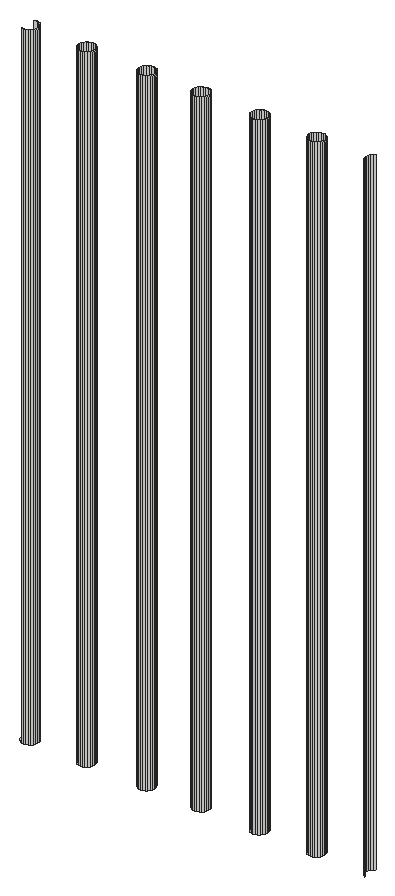
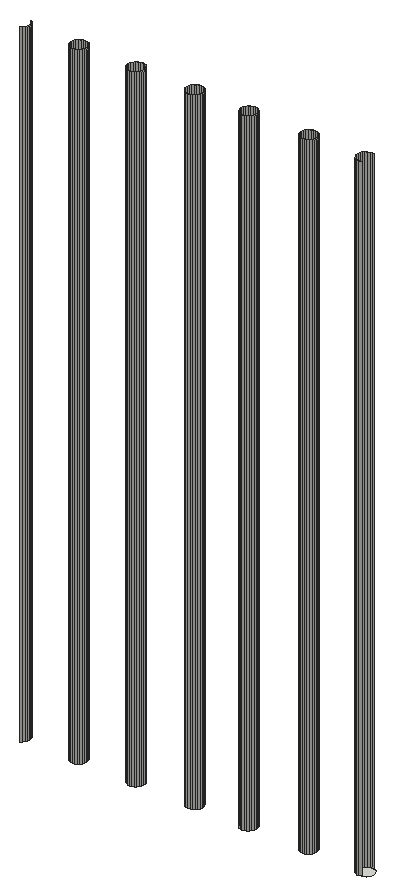
# SketchUp Ruby script. Lengths in inches.
U = 1.inch
M = Sketchup.active_model
def pt(a) = Geom::Point3d.new(a.map { |v| v * U })
def face(e, loops, mat)
  f = e.add_face(loops[0].map { |a| pt(a) })
  loops[1..].each { |l| e.add_face(l.map { |a| pt(a) }).erase! }
  f.material = f.back_material = mat if mat
  f
end
# faces: each face lists its corners as indices into pts; further lists are holes
def faces(e, pts, list, mat = nil) = list.each { |f| face(e, (f[0].is_a?(Array) ? f : [f]).map { |l| l.map { |i| pts[i] } }, mat) }
# xy, xz, yz: faces in a plane at the given z, y or x. An outline is a flat list of corners, or four numbers for a rectangle; further outlines are holes
def ring(l) = l.size == 4 ? [[l[0], l[1]], [l[2], l[1]], [l[2], l[3]], [l[0], l[3]]] : l.each_slice(2).to_a
def flat(e, list, mat, &to3) = list.each { |f| face(e, (f[0].is_a?(Array) ? f : [f]).map { |l| ring(l).map { |u, v| to3.(u, v) } }, mat) }
def xy(e, z, list, mat = nil) = flat(e, list, mat) { |x, y| [x, y, z] }
def xz(e, y, list, mat = nil) = flat(e, list, mat) { |x, z| [x, y, z] }
def yz(e, x, list, mat = nil) = flat(e, list, mat) { |y, z| [x, y, z] }
def lines(e, pts, list) = list.each { |a, b| e.add_line(pt(pts[a]), pt(pts[b])) }
# prism: a flat outline (further loops are holes) pulled along v
def prism(e, loops, v, mat = nil)
  f = face(e, loops, mat); d = Geom::Vector3d.new(v.map { |x| x * U })
  f.pushpull(f.normal.samedirection?(d) ? d.length : -d.length)
end
def box(e, o, s, mat = nil) = prism(e, [[o, [o[0] + s[0], o[1], o[2]], [o[0] + s[0], o[1] + s[1], o[2]], [o[0], o[1] + s[1], o[2]]]], [0, 0, s[2]], mat)
def at(x, y, z, deg = 0) = Geom::Transformation.translation(pt([x, y, z])) * Geom::Transformation.rotation(ORIGIN, Z_AXIS, deg.degrees)
def axes(o, x, y, z) = Geom::Transformation.new([*x, 0, *y, 0, *z, 0, *pt(o).to_a, 1])
def part(name) = M.definitions.add(name)
# library, detail: a bought-in or finely detailed component or shape, given as its bounding box
def library(name, o, s) = part(name).tap { |d| box(d.entities, o, s) }
def detail(e, o, s) = box(e.add_group.entities, o, s)
def put(e, d, t, mat = nil) = e.add_instance(d, t).tap { |i| i.material = mat if mat }
def group(e, t, mat = nil) = e.add_group.tap { |g| g.transformation = t; g.material = mat if mat }.entities
root = M.entities
xy(root,614.8125,[[418.54,132.04,418.33,132.07,418.14,132.15,417.97,132.28,417.84,132.45,417.76,132.64,417.73,132.85,417.76,133.06,417.84,133.26,417.97,133.43,418.14,133.56,418.33,133.64,418.54,133.67,418.75,133.64,418.95,133.56,419.12,133.43,419.25,133.26,419.33,133.06,419.36,132.85,419.33,132.64,419.25,132.45,419.12,132.28,418.95,132.15,418.75,132.07],[424.36,132.04,424.14,132.07,423.95,132.15,423.78,132.28,423.65,132.45,423.57,132.64,423.54,132.85,423.57,133.06,423.65,133.26,423.78,133.43,423.95,133.56,424.14,133.64,424.36,133.67,424.57,133.64,424.76,133.56,424.93,133.43,425.06,133.26,425.14,133.06,425.17,132.85,425.14,132.64,425.06,132.45,424.93,132.28,424.76,132.15,424.57,132.07],[430.54,132.04,430.33,132.07,430.14,132.15,429.97,132.28,429.84,132.45,429.76,132.64,429.73,132.85,429.76,133.06,429.84,133.26,429.97,133.43,430.14,133.56,430.33,133.64,430.54,133.67,430.75,133.64,430.95,133.56,431.12,133.43,431.25,133.26,431.33,133.06,431.36,132.85,431.33,132.64,431.25,132.45,431.12,132.28,430.95,132.15,430.75,132.07],[436.11,132.04,435.89,132.07,435.7,132.15,435.53,132.28,435.4,132.45,435.32,132.64,435.29,132.85,435.32,133.06,435.4,133.26,435.53,133.43,435.7,133.56,435.89,133.64,436.11,133.67,436.32,133.64,436.51,133.56,436.68,133.43,436.81,133.26,436.89,133.06,436.92,132.85,436.89,132.64,436.81,132.45,436.68,132.28,436.51,132.15,436.32,132.07],[442.11,132.04,441.89,132.07,441.7,132.15,441.53,132.28,441.4,132.45,441.32,132.64,441.29,132.85,441.32,133.06,441.4,133.26,441.53,133.43,441.7,133.56,441.89,133.64,442.11,133.67,442.32,133.64,442.51,133.56,442.68,133.43,442.81,133.26,442.89,133.06,442.92,132.85,442.89,132.64,442.81,132.45,442.68,132.28,442.51,132.15,442.32,132.07],
  [447.98,132.04,447.77,132.07,447.57,132.15,447.41,132.28,447.28,132.45,447.2,132.64,447.17,132.85,447.2,133.06,447.28,133.26,447.41,133.43,447.57,133.56,447.77,133.64,447.98,133.67,448.19,133.64,448.39,133.56,448.55,133.43,448.68,133.26,448.77,133.06,448.79,132.85,448.77,132.64,448.68,132.45,448.55,132.28,448.39,132.15,448.19,132.07]])
p = [[418.33,132.07,614.8125],[418.54,132.04,614.8125],[418.54,132.04,680.58],[418.33,132.07,680.58],[418.75,132.07,614.8125],[418.75,132.07,680.58],
  [424.14,132.07,614.8125],[424.36,132.04,614.8125],[424.36,132.04,680.58],[424.14,132.07,680.58],[424.57,132.07,614.8125],[424.57,132.07,680.58],
  [430.33,132.07,614.8125],[430.54,132.04,614.8125],[430.54,132.04,680.58],[430.33,132.07,680.58],[430.75,132.07,614.8125],[430.75,132.07,680.58],
  [435.89,132.07,614.8125],[436.11,132.04,614.8125],[436.11,132.04,680.58],[435.89,132.07,680.58],[436.32,132.07,614.8125],[436.32,132.07,680.58],
  [441.89,132.07,614.8125],[442.11,132.04,614.8125],[442.11,132.04,680.58],[441.89,132.07,680.58],[442.32,132.07,614.8125],[442.32,132.07,680.58],
  [447.77,132.07,614.8125],[447.98,132.04,614.8125],[447.98,132.04,680.58],[447.77,132.07,680.58],[448.19,132.07,614.8125],[448.19,132.07,680.58],
  [418.95,132.15,614.8125],[418.95,132.15,680.58],[423.95,132.15,614.8125],[423.95,132.15,680.58],[424.76,132.15,614.8125],[424.76,132.15,680.58],
  [430.14,132.15,614.8125],[430.14,132.15,680.58],[430.95,132.15,614.8125],[430.95,132.15,680.58],[435.7,132.15,614.8125],[435.7,132.15,680.58],
  [436.51,132.15,614.8125],[436.51,132.15,680.58],[441.7,132.15,614.8125],[441.7,132.15,680.58],[442.51,132.15,614.8125],[442.51,132.15,680.58],
  [447.57,132.15,614.8125],[447.57,132.15,680.58],[448.39,132.15,614.8125],[448.39,132.15,680.58],[419.12,132.28,614.8125],[419.12,132.28,680.58],
  [423.78,132.28,614.8125],[423.78,132.28,680.58],[424.93,132.28,614.8125],[424.93,132.28,680.58],[429.97,132.28,614.8125],[429.97,132.28,680.58],
  [431.12,132.28,614.8125],[431.12,132.28,680.58],[435.53,132.28,614.8125],[435.53,132.28,680.58],[436.68,132.28,614.8125],[436.68,132.28,680.58],
  [441.53,132.28,614.8125],[441.53,132.28,680.58],[442.68,132.28,614.8125],[442.68,132.28,680.58],[447.41,132.28,614.8125],[447.41,132.28,680.58],
  [448.55,132.28,614.8125],[448.55,132.28,680.58],[453.28,132.28,614.8125],[453.45,132.15,614.8125],[453.45,132.15,680.58],[453.28,132.28,680.58],
  [419.25,132.45,614.8125],[419.25,132.45,680.58],[423.65,132.45,614.8125],[423.65,132.45,680.58],[425.06,132.45,614.8125],[425.06,132.45,680.58],
  [429.84,132.45,614.8125],[429.84,132.45,680.58],[431.25,132.45,614.8125],[431.25,132.45,680.58],[435.4,132.45,614.8125],[435.4,132.45,680.58],
  [436.81,132.45,614.8125],[436.81,132.45,680.58],[441.4,132.45,614.8125],[441.4,132.45,680.58],[442.81,132.45,614.8125],[442.81,132.45,680.58],
  [447.28,132.45,614.8125],[447.28,132.45,680.58],[448.68,132.45,614.8125],[448.68,132.45,680.58],[453.15,132.45,614.8125],[453.15,132.45,680.58],
  [419.33,132.64,614.8125],[419.33,132.64,680.58],[423.57,132.64,614.8125],[423.57,132.64,680.58],[425.14,132.64,614.8125],[425.14,132.64,680.58],
  [429.76,132.64,614.8125],[429.76,132.64,680.58],[431.33,132.64,614.8125],[431.33,132.64,680.58],[435.32,132.64,614.8125],[435.32,132.64,680.58],
  [436.89,132.64,614.8125],[436.89,132.64,680.58],[441.32,132.64,614.8125],[441.32,132.64,680.58],[442.89,132.64,614.8125],[442.89,132.64,680.58],
  [447.2,132.64,614.8125],[447.2,132.64,680.58],[448.77,132.64,614.8125],[448.77,132.64,680.58],[453.07,132.64,614.8125],[453.07,132.64,680.58],
  [419.36,132.85,614.8125],[419.36,132.85,680.58],[423.54,132.85,614.8125],[423.54,132.85,680.58],[425.17,132.85,614.8125],[425.17,132.85,680.58],
  [429.73,132.85,614.8125],[429.73,132.85,680.58],[431.36,132.85,614.8125],[431.36,132.85,680.58],[435.29,132.85,614.8125],[435.29,132.85,680.58],
  [436.92,132.85,614.8125],[436.92,132.85,680.58],[441.29,132.85,614.8125],[441.29,132.85,680.58],[442.92,132.85,614.8125],[442.92,132.85,680.58],
  [447.17,132.85,614.8125],[447.17,132.85,680.58],[448.79,132.85,614.8125],[448.79,132.85,680.58],[453.04,132.85,614.8125],[453.04,132.85,680.58],
  [419.33,133.06,614.8125],[419.33,133.06,680.58],[423.57,133.06,614.8125],[423.57,133.06,680.58],[425.14,133.06,614.8125],[425.14,133.06,680.58],
  [429.76,133.06,614.8125],[429.76,133.06,680.58],[431.33,133.06,614.8125],[431.33,133.06,680.58],[435.32,133.06,614.8125],[435.32,133.06,680.58],
  [436.89,133.06,614.8125],[436.89,133.06,680.58],[441.32,133.06,614.8125],[441.32,133.06,680.58],[442.89,133.06,614.8125],[442.89,133.06,680.58],
  [447.2,133.06,614.8125],[447.2,133.06,680.58],[448.77,133.06,614.8125],[448.77,133.06,680.58],[453.07,133.06,614.8125],[453.07,133.06,680.58],
  [419.25,133.26,614.8125],[419.25,133.26,680.58],[423.65,133.26,614.8125],[423.65,133.26,680.58],[425.06,133.26,614.8125],[425.06,133.26,680.58],
  [429.84,133.26,614.8125],[429.84,133.26,680.58],[431.25,133.26,614.8125],[431.25,133.26,680.58],[435.4,133.26,614.8125],[435.4,133.26,680.58],
  [436.81,133.26,614.8125],[436.81,133.26,680.58],[441.4,133.26,614.8125],[441.4,133.26,680.58],[442.81,133.26,614.8125],[442.81,133.26,680.58],
  [447.28,133.26,614.8125],[447.28,133.26,680.58],[448.68,133.26,614.8125],[448.68,133.26,680.58],[453.15,133.26,614.8125],[453.15,133.26,680.58],
  [419.12,133.43,614.8125],[419.12,133.43,680.58],[423.78,133.43,614.8125],[423.78,133.43,680.58],[424.93,133.43,614.8125],[424.93,133.43,680.58],
  [429.97,133.43,614.8125],[429.97,133.43,680.58],[431.12,133.43,614.8125],[431.12,133.43,680.58],[435.53,133.43,614.8125],[435.53,133.43,680.58],
  [436.68,133.43,614.8125],[436.68,133.43,680.58],[441.53,133.43,614.8125],[441.53,133.43,680.58],[442.68,133.43,614.8125],[442.68,133.43,680.58],
  [447.41,133.43,614.8125],[447.41,133.43,680.58],[448.55,133.43,614.8125],[448.55,133.43,680.58],[453.28,133.43,614.8125],[453.28,133.43,680.58],
  [418.95,133.56,614.8125],[418.95,133.56,680.58],[423.95,133.56,614.8125],[423.95,133.56,680.58],[424.76,133.56,614.8125],[424.76,133.56,680.58],
  [430.14,133.56,614.8125],[430.14,133.56,680.58],[430.95,133.56,614.8125],[430.95,133.56,680.58],[435.7,133.56,614.8125],[435.7,133.56,680.58],
  [436.51,133.56,614.8125],[436.51,133.56,680.58],[441.7,133.56,614.8125],[441.7,133.56,680.58],[442.51,133.56,614.8125],[442.51,133.56,680.58],
  [447.57,133.56,614.8125],[447.57,133.56,680.58],[448.39,133.56,614.8125],[448.39,133.56,680.58],[453.45,133.56,614.8125],[453.45,133.56,680.58],
  [418.54,133.67,614.8125],[418.33,133.64,614.8125],[418.33,133.64,680.58],[418.54,133.67,680.58],[418.75,133.64,614.8125],[418.75,133.64,680.58],
  [424.14,133.64,614.8125],[424.14,133.64,680.58],[424.36,133.67,614.8125],[424.36,133.67,680.58],[424.57,133.64,614.8125],[424.57,133.64,680.58],
  [430.33,133.64,614.8125],[430.33,133.64,680.58],[430.54,133.67,614.8125],[430.54,133.67,680.58],[430.75,133.64,614.8125],[430.75,133.64,680.58],
  [435.89,133.64,614.8125],[435.89,133.64,680.58],[436.11,133.67,614.8125],[436.11,133.67,680.58],[436.32,133.64,614.8125],[436.32,133.64,680.58],
  [441.89,133.64,614.8125],[441.89,133.64,680.58],[442.11,133.67,614.8125],[442.11,133.67,680.58],[442.32,133.64,614.8125],[442.32,133.64,680.58],
  [447.77,133.64,614.8125],[447.77,133.64,680.58],[447.98,133.67,614.8125],[447.98,133.67,680.58],[448.19,133.64,614.8125],[448.19,133.64,680.58],
  [447.88,132.57,680.58],[447.88,132.57,614.8125],[442.01,132.57,680.58],[442.01,132.57,614.8125],[436.13,132.57,680.58],[436.13,132.57,614.8125],
  [430.26,132.57,680.58],[430.26,132.57,614.8125],[424.38,132.57,680.58],[424.38,132.57,614.8125],[418.51,132.57,680.58],[418.51,132.57,614.8125]]
faces(root,p,[[0,1,2,3],[1,4,5,2],[6,7,8,9],[7,10,11,8],[12,13,14,15],[13,16,17,14],[18,19,20,21],[19,22,23,20],
  [24,25,26,27],[25,28,29,26],[30,31,32,33],[31,34,35,32],[4,36,37,5],[38,6,9,39],[10,40,41,11],[42,12,15,43],
  [16,44,45,17],[46,18,21,47],[22,48,49,23],[50,24,27,51],[28,52,53,29],[54,30,33,55],[34,56,57,35],[36,58,59,37],
  [60,38,39,61],[40,62,63,41],[64,42,43,65],[44,66,67,45],[68,46,47,69],[48,70,71,49],[72,50,51,73],[52,74,75,53],
  [76,54,55,77],[56,78,79,57],[80,81,82,83],[58,84,85,59],[86,60,61,87],[62,88,89,63],[90,64,65,91],[66,92,93,67],
  [94,68,69,95],[70,96,97,71],[98,72,73,99],[74,100,101,75],[102,76,77,103],[78,104,105,79],[106,80,83,107],[84,108,109,85],
  [110,86,87,111],[88,112,113,89],[114,90,91,115],[92,116,117,93],[118,94,95,119],[96,120,121,97],[122,98,99,123],[100,124,125,101],
  [126,102,103,127],[104,128,129,105],[130,106,107,131],[108,132,133,109],[134,110,111,135],[112,136,137,113],[138,114,115,139],[116,140,141,117],
  [142,118,119,143],[120,144,145,121],[146,122,123,147],[124,148,149,125],[150,126,127,151],[128,152,153,129],[154,130,131,155],[132,156,157,133],
  [158,134,135,159],[136,160,161,137],[162,138,139,163],[140,164,165,141],[166,142,143,167],[144,168,169,145],[170,146,147,171],[148,172,173,149],
  [174,150,151,175],[152,176,177,153],[178,154,155,179],[156,180,181,157],[182,158,159,183],[160,184,185,161],[186,162,163,187],[164,188,189,165],
  [190,166,167,191],[168,192,193,169],[194,170,171,195],[172,196,197,173],[198,174,175,199],[176,200,201,177],[202,178,179,203],[180,204,205,181],
  [206,182,183,207],[184,208,209,185],[210,186,187,211],[188,212,213,189],[214,190,191,215],[192,216,217,193],[218,194,195,219],[196,220,221,197],
  [222,198,199,223],[200,224,225,201],[226,202,203,227],[204,228,229,205],[230,206,207,231],[208,232,233,209],[234,210,211,235],[212,236,237,213],
  [238,214,215,239],[216,240,241,217],[242,218,219,243],[220,244,245,221],[246,222,223,247],[224,248,249,225],[250,226,227,251],[252,253,254,255],
  [256,252,255,257],[228,256,257,229],[258,230,231,259],[260,258,259,261],[262,260,261,263],[232,262,263,233],[264,234,235,265],[266,264,265,267],
  [268,266,267,269],[236,268,269,237],[270,238,239,271],[272,270,271,273],[274,272,273,275],[240,274,275,241],[276,242,243,277],[278,276,277,279],
  [280,278,279,281],[244,280,281,245],[282,246,247,283],[284,282,283,285],[286,284,285,287],[248,286,287,249]])
lines(root,p,[[288,289],[290,291],[292,293],[294,295],[296,297],[298,299]])
